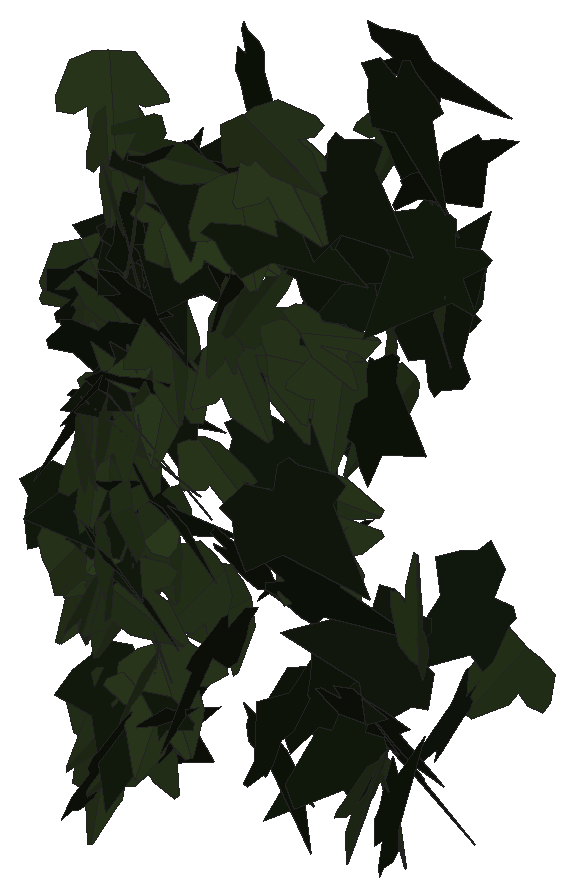
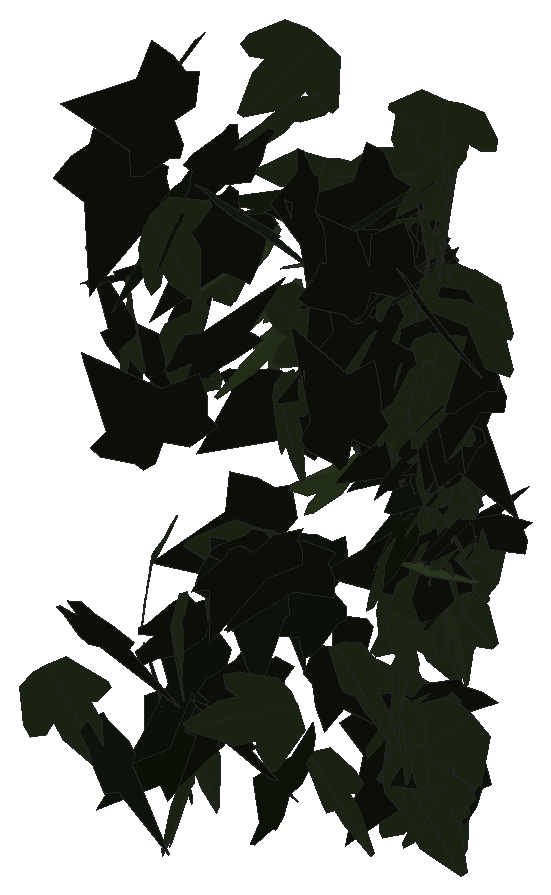
# SketchUp Ruby script. Lengths in inches.
U = 1.inch
M = Sketchup.active_model
def pt(a) = Geom::Point3d.new(a.map { |v| v * U })
def face(e, loops, mat)
  f = e.add_face(loops[0].map { |a| pt(a) })
  loops[1..].each { |l| e.add_face(l.map { |a| pt(a) }).erase! }
  f.material = f.back_material = mat if mat
  f
end
# faces: each face lists its corners as indices into pts; further lists are holes
def faces(e, pts, list, mat = nil) = list.each { |f| face(e, (f[0].is_a?(Array) ? f : [f]).map { |l| l.map { |i| pts[i] } }, mat) }
# xy, xz, yz: faces in a plane at the given z, y or x. An outline is a flat list of corners, or four numbers for a rectangle; further outlines are holes
def ring(l) = l.size == 4 ? [[l[0], l[1]], [l[2], l[1]], [l[2], l[3]], [l[0], l[3]]] : l.each_slice(2).to_a
def flat(e, list, mat, &to3) = list.each { |f| face(e, (f[0].is_a?(Array) ? f : [f]).map { |l| ring(l).map { |u, v| to3.(u, v) } }, mat) }
def xy(e, z, list, mat = nil) = flat(e, list, mat) { |x, y| [x, y, z] }
def xz(e, y, list, mat = nil) = flat(e, list, mat) { |x, z| [x, y, z] }
def yz(e, x, list, mat = nil) = flat(e, list, mat) { |y, z| [x, y, z] }
def lines(e, pts, list) = list.each { |a, b| e.add_line(pt(pts[a]), pt(pts[b])) }
# prism: a flat outline (further loops are holes) pulled along v
def prism(e, loops, v, mat = nil)
  f = face(e, loops, mat); d = Geom::Vector3d.new(v.map { |x| x * U })
  f.pushpull(f.normal.samedirection?(d) ? d.length : -d.length)
end
def box(e, o, s, mat = nil) = prism(e, [[o, [o[0] + s[0], o[1], o[2]], [o[0] + s[0], o[1] + s[1], o[2]], [o[0], o[1] + s[1], o[2]]]], [0, 0, s[2]], mat)
def at(x, y, z, deg = 0) = Geom::Transformation.translation(pt([x, y, z])) * Geom::Transformation.rotation(ORIGIN, Z_AXIS, deg.degrees)
def axes(o, x, y, z) = Geom::Transformation.new([*x, 0, *y, 0, *z, 0, *pt(o).to_a, 1])
def part(name) = M.definitions.add(name)
# library, detail: a bought-in or finely detailed component or shape, given as its bounding box
def library(name, o, s) = part(name).tap { |d| box(d.entities, o, s) }
def detail(e, o, s) = box(e.add_group.entities, o, s)
def put(e, d, t, mat = nil) = e.add_instance(d, t).tap { |i| i.material = mat if mat }
def group(e, t, mat = nil) = e.add_group.tap { |g| g.transformation = t; g.material = mat if mat }.entities
root = M.entities
M.materials.add("efeu1").color = [18, 25, 13]
M.materials.add("efeu2").color = [43, 57, 29]
c1 = part("ivyleaf_10")
p = [[0,0.5,-0.03],[-0.0625,2.02,-0.43],[-0.19,2.01,-0.46],[-0.54,1.05,-0.29],[-0.52,0.625,-0.18],[-0.83,0.76,-0.28],
  [-1.16,0.64,-0.33],[-1.15,0.33,-0.24],[-0.77,-0.39,0.02],[-0.3,-0.51,0.16],[0.04,-0.48,0.23],[-0.02,2.01,-0.4375],
  [-0.06,2.01,-0.43],[0.04,-0.49,0.23],[0.67,-0.49,0.14],[1.38,0.36,-0.2],[1.375,0.51,-0.24],[0.81,0.65,-0.19],
  [0.62,0.59,-0.15],[0.6,1.09,-0.28],[0.5,1.23,-0.31]]
faces(c1.entities,p,[[0,1,2,3,4,5,6,7,8,9,10],[11,12,0,13,14,15,16,17,18,19,20]],"efeu2")
c2 = part("ivyleaf_9")
p = [[1.54,2.16,1.25],[1.36,2.04,1.19],[-0.21,0.99,0.68],[-0.71,1.11,0.82],[-0.85,0.86,0.67],[-0.8,0.17,0.21],
  [-0.9,-0.01,0.1],[-0.67,-0.16,-0.02],[-0.08,-0.08,-0.05],[-0.03,-0.6,-0.4],[0.65,-0.88,-0.66],[0.83,-0.6,-0.49],
  [1.29,-0.42,-0.43],[1.8125,-0.07,-0.26],[1.21,0.44,0.15]]
faces(c2.entities,p,[[0,1,2,3,4,5,6,7,8,9,10,11,12,13,14]],"efeu1")
put(root,c1,axes([46.82,223.79,215.375],[0.30689,-0.17648,-0.35309],[-0.31194,0.16564,-0.35392],[0.24189,0.43752,-0.00843]))
put(root,c2,axes([46.77,221.68,218.99],[-0.26591,0.32248,-0.27441],[0.12873,-0.24713,-0.41516],[-0.40339,-0.29144,0.0484]))
put(root,c1,axes([46.61,221.95,214.38],[0.06345,0.46426,-0.17446],[-0.06333,-0.16686,-0.46706],[-0.4919,0.08136,0.03763]))
put(root,c1,axes([46.6875,221.47,218.47],[-0.1604,0.43532,0.18647],[-0.13321,0.14746,-0.45881],[-0.45445,-0.19687,0.06867]))
put(root,c1,axes([46.83,222.19,214.4375],[0.37847,0.13915,-0.29563],[-0.32579,0.1261,-0.35772],[-0.02499,0.4634,0.18612]))
put(root,c1,axes([46.64,222.06,219.93],[-0.15553,-0.44023,-0.1789],[0.0777,0.16215,-0.46655],[0.4688,-0.17293,0.01797]))
put(root,c1,axes([46.58,221.66,220.17],[-0.44765,-0.1511,-0.16364],[0.16974,0.0064,-0.47026],[0.14421,-0.47658,0.04557]))
put(root,c1,axes([46.58,221.19,217.02],[0.06755,0.12705,-0.47885],[0.14684,0.45643,0.14181],[0.47315,-0.15979,0.02435]))
put(root,c1,axes([46.73,221.78,216.78],[0.16694,0.38069,-0.27786],[-0.18616,-0.21755,-0.4099],[-0.43298,0.24031,0.0691]))
put(root,c2,axes([47.07,221.99,220.55],[-0.28103,0.2768,0.30725],[-0.21871,0.21579,-0.39446],[-0.35098,-0.35611,-0.00021]))
put(root,c1,axes([46.79,221.57,216.68],[0.12726,-0.4742,-0.09455],[-0.03702,0.08792,-0.49081],[0.48211,0.13192,-0.01273]))
put(root,c1,axes([46.6875,221.69,218.05],[0.11882,0.46479,-0.14089],[-0.04843,-0.13298,-0.47955],[-0.48326,0.12761,0.01342]))
put(root,c1,axes([46.78,222.07,219.12],[0.03325,0.46398,-0.18335],[-0.00464,0.18403,0.46488],[0.49887,-0.02921,0.01654]))
put(root,c1,axes([47.08,221.625,217.54],[-0.23958,0.12458,0.42081],[-0.4336,0.00683,-0.24888],[-0.06776,-0.48418,0.10476]))
put(root,c2,axes([46.77,222,217.32],[0.10972,-0.3803,-0.30551],[0.08778,-0.29264,0.3958],[-0.47985,-0.14049,0.00254]))
put(root,c2,axes([46.5,221.61,217.73],[-0.04451,-0.36504,-0.33877],[0.22637,0.28812,-0.34021],[0.44359,-0.18366,0.13962]))
put(root,c2,axes([46.42,221.64,219.87],[0.27297,0.05631,0.41511],[0.3965,0.12515,-0.27771],[-0.13518,0.4808,0.02367]))
put(root,c2,axes([46.79,221.58,219.6],[0.34529,0.32059,-0.16733],[-0.13687,-0.09829,-0.47075],[-0.33473,0.37089,0.01988]))
put(root,c1,axes([46.7,221.54,220.52],[-0.42496,-0.19869,-0.17301],[0.18869,-0.00038,-0.46303],[0.18387,-0.45883,0.0753]))
put(root,c1,axes([46.77,222.03,214.97],[0.01467,-0.18184,0.46553],[0.08905,-0.45733,-0.18144],[0.49179,0.08823,0.01897]))
put(root,c1,axes([46.57,221.89,215.19],[-0.26759,-0.1951,-0.37461],[0.35309,0.14004,-0.32514],[0.23179,-0.43855,0.06283]))
put(root,c1,axes([46.91,222.01,217.02],[0.08621,0.19271,-0.45324],[-0.2035,-0.40508,-0.21094],[-0.4485,0.22084,0.00859]))
put(root,c1,axes([46.77,222.49,216.79],[0.11328,-0.30008,0.38357],[0.11296,-0.36688,-0.32038],[0.47372,0.15924,-0.01533]))
put(root,c1,axes([47.18,221.76,218.17],[0.07671,-0.01508,-0.49385],[-0.44837,0.20781,-0.07599],[0.20755,0.45452,0.01836]))
put(root,c1,axes([46.93,221.7,218.74],[-0.01928,0.46785,0.17534],[-0.18986,0.15545,-0.43565],[-0.46215,-0.08338,0.17166]))
put(root,c2,axes([46.83,222.39,218.76],[0.13338,-0.32118,-0.35924],[0.14471,-0.32884,0.34774],[-0.45964,-0.19674,0.00524]))
put(root,c1,axes([47.04,221.57,218.74],[0.35221,-0.16904,-0.31205],[-0.2773,0.14328,-0.39061],[0.22147,0.44822,0.00718]))
put(root,c1,axes([46.83,221.84,217.07],[0.41424,-0.26825,-0.08031],[0.00776,0.15435,-0.47552],[0.27991,0.39271,0.13203]))
put(root,c1,axes([46.9,222.13,217.24],[-0.49845,-0.02607,0.0295],[0.02483,-0.49892,-0.0214],[0.03055,-0.01987,0.49867]))
put(root,c1,axes([46.96,221.89,216.61],[-0.13131,-0.44619,0.18351],[-0.03547,-0.18074,-0.46484],[0.48115,-0.13509,0.01581]))
put(root,c1,axes([46.98,221.45,221.65],[-0.33317,0.34293,0.1463],[-0.13314,0.07383,-0.47626],[-0.34824,-0.3563,0.04212]))
put(root,c2,axes([46.99,221.2,214.56],[-0.15844,0.29308,-0.37283],[-0.20139,0.3143,0.33265],[0.42934,0.25558,0.01845]))
put(root,c1,axes([47.01,222.17,215.93],[-0.33606,0.34989,0.121],[-0.08049,0.09046,-0.48512],[-0.36136,-0.34554,-0.00447]))
put(root,c1,axes([47.04,222.03,219.15],[0.03664,0.15212,-0.47489],[-0.02414,0.47615,0.15066],[0.49807,0.01189,0.04224]))
put(root,c1,axes([47.12,221.25,216.875],[-0.02583,0.10493,-0.48818],[-0.10809,0.47607,0.10804],[0.48749,0.11112,-0.00191]))
put(root,c1,axes([46.85,221.62,222.72],[0.46319,0.1612,0.09729],[0.08762,0.04414,-0.49028],[-0.16666,0.47124,0.01265]))
put(root,c1,axes([46.93,221.66,222.08],[0.0206,0.47589,-0.15201],[-0.00834,-0.15179,-0.47633],[-0.49951,0.02216,0.00169]))
put(root,c1,axes([47.04,222.14,214.74],[0.01557,-0.25413,0.43032],[0.01222,-0.43021,-0.2545],[0.49961,0.01844,-0.00718]))
put(root,c2,axes([46.63,221.89,217.33],[0.38798,0.01259,0.31514],[0.31157,0.06229,-0.38606],[-0.04898,0.49595,0.04048]))
put(root,c2,axes([46.68,223.57,219.62],[-0.02299,-0.09481,0.49039],[0.36286,-0.34051,-0.04882],[0.34322,0.35364,0.08446]))
put(root,c1,axes([47.25,225.875,217.92],[-0.03166,0.05115,-0.49637],[-0.23881,0.43516,0.06007],[0.43814,0.24088,-0.00313]))
put(root,c1,axes([47.12,222.04,215.56],[0.10552,-0.44612,-0.19962],[-0.05205,0.1928,-0.45839],[0.48596,0.11751,-0.00575]))
put(root,c2,axes([46.71,221.7,217.04],[0.36429,-0.31913,0.1243],[0.09979,-0.07469,-0.48421],[0.32763,0.37759,0.00927]))
put(root,c1,axes([47.22,222.85,216.21],[0.37723,-0.17084,-0.2802],[-0.25699,0.11171,-0.4141],[0.2041,0.45643,-0.00353]))
put(root,c2,axes([46.79,221.62,218.89],[0.44913,0.12155,0.18306],[0.15945,0.10635,-0.46181],[-0.1512,0.4732,0.05676]))
put(root,c1,axes([47.1,221.64,220.94],[-0.29958,0.39759,0.04665],[-0.05124,0.0197,-0.49698],[-0.39702,-0.30255,0.02894]))
put(root,c2,axes([47.07,221.9,215.41],[-0.2799,-0.40493,-0.08769],[0.05211,0.07058,-0.49224],[0.41102,-0.2847,0.00269]))
put(root,c1,axes([47.07,222.01,220.19],[-0.07306,-0.15963,-0.46817],[0.17446,0.43452,-0.17538],[0.46285,-0.18898,-0.0078]))
put(root,c1,axes([46.98,221.58,216.61],[-0.30475,-0.20215,-0.34097],[0.30985,0.14677,-0.36394],[0.24723,-0.43312,0.03582]))
put(root,c1,axes([46.99,221.84,221.42],[0.3706,-0.23549,0.23916],[0.20527,-0.12286,-0.43906],[0.26555,0.42361,0.00561]))
put(root,c2,axes([46.91,222.16,217.81],[0.38681,-0.31542,0.02987],[0.01646,-0.02706,-0.499],[0.3164,0.38701,-0.01055]))
put(root,c1,axes([46.89,224.65,216.54],[-0.16502,-0.06552,-0.46741],[0.45476,0.11048,-0.17604],[0.12635,-0.48322,0.02313]))
put(root,c2,axes([47.0625,221.99,220.71],[0.08964,-0.44345,-0.21287],[-0.04873,0.20731,-0.45238],[0.48948,0.10185,-0.00606]))
put(root,c1,axes([47.13,222.1875,217.26],[0.01903,-0.49963,0.00328],[0.18506,0.004,-0.46447],[0.4641,0.01889,0.18508]))
put(root,c2,axes([47.1875,221.74,214.79],[0.25418,0.40568,0.14428],[0.07424,0.12374,-0.47872],[-0.42413,0.26478,0.00267]))
put(root,c2,axes([47.03,221.4,220.34],[0.49698,0.04863,-0.02548],[-0.02536,-0.00248,-0.49935],[-0.04869,0.49762,0]))
put(root,c2,axes([46.84,221.84,218.34],[0.21613,-0.31536,0.32223],[0.30304,-0.16299,-0.36277],[0.33385,0.35211,0.12068]))
put(root,c1,axes([47.28,222.13,219.25],[0.11303,-0.48643,-0.0247],[-0.00136,0.02504,-0.49937],[0.48705,0.11295,0.00434]))
put(root,c2,axes([47.21,221.77,220.65],[-0.06908,-0.11012,0.48281],[0.27459,0.39716,0.12987],[-0.4121,0.28309,0.0056]))
put(root,c2,axes([47.11,222.17,219.19],[0.06506,-0.4642,-0.17402],[-0.02469,0.17226,-0.46874],[0.49513,0.06959,-0.00051]))
put(root,c2,axes([46.99,222.53,220.21],[0.47448,0.05094,0.14923],[0.1496,0.00416,-0.47708],[-0.04985,0.49738,-0.01129]))
put(root,c1,axes([47.22,222.08,215.13],[-0.24468,-0.26366,0.34729],[0.23603,-0.41494,-0.14872],[0.36663,0.09117,0.32752]))
put(root,c2,axes([47.0625,221.62,218.72],[0.46036,-0.19434,0.0175],[0.01655,-0.0058,-0.49969],[0.19442,0.46065,0.00109]))
put(root,c2,axes([47.2,224.62,218.36],[0.04208,-0.42382,-0.26193],[-0.02957,0.26028,-0.42589],[0.49735,0.05133,-0.00316]))
put(root,c2,axes([47.18,221.76,221.01],[0.04444,0.03877,-0.49651],[0.05402,0.49517,0.0435],[0.49508,-0.0575,0.03982]))
put(root,c1,axes([47.29,222.09,219.07],[-0.24222,-0.35782,0.25159],[0.23431,-0.34899,-0.27076],[0.36937,-0.01327,0.33674]))
put(root,c2,axes([47.21,222.58,220.84],[-0.15698,-0.07507,0.46874],[0.46812,0.05757,0.16599],[-0.0789,0.49097,0.05221]))
put(root,c1,axes([47.33,222.2,221.1],[-0.13752,-0.38235,0.29136],[0.19858,-0.32117,-0.32774],[0.43778,0.02557,0.24019]))
put(root,c1,axes([47.25,222,215.55],[0.38898,0.24821,0.19258],[0.16302,0.10252,-0.46143],[-0.26855,0.42176,-0.00118]))
put(root,c2,axes([47.23,222.18,221.67],[0.01862,-0.48418,0.12339],[0.18798,-0.10762,-0.45064],[0.46294,0.06318,0.17803]))
put(root,c2,axes([47.31,222.19,220.52],[-0.13756,-0.38111,0.29297],[0.19861,-0.32256,-0.32635],[0.43776,0.02659,0.24013]))
put(root,c1,axes([47.17,221.66,221.87],[0.09736,-0.08169,0.48358],[0.39188,0.30939,-0.02664],[-0.29488,0.38419,0.12427]))
put(root,c1,axes([47.39,221.97,219.68],[-0.01774,-0.48976,0.09909],[0.23773,-0.09548,-0.42938],[0.43951,0.03187,0.23625]))
put(root,c2,axes([47.23,223.51,222.21],[0.04571,-0.04238,-0.4961],[0.4979,0.00138,0.04576],[-0.00251,-0.4982,0.04233]))
put(root,c2,axes([47.25,221.99,221.42],[0.29116,0.01323,0.40626],[0.39058,0.1293,-0.28413],[-0.11258,0.48281,0.06496]))
put(root,c2,axes([47.81,222.41,215.98],[-0.2064,0.24126,-0.38626],[0.22689,-0.31322,-0.31688],[-0.39487,-0.30608,0.01982]))
put(root,c2,axes([47.62,223.65,217.83],[-0.1407,-0.30014,-0.37433],[0.18129,0.32792,-0.33107],[0.44423,-0.22888,0.01655]))
put(root,c1,axes([48.05,222.98,219.28],[0.24265,-0.13176,-0.41685],[-0.25565,0.34397,-0.25754],[0.35463,0.33812,0.09956]))
put(root,c2,axes([48.09,222.15,220.47],[-0.06248,0.05533,-0.49299],[-0.40006,0.28819,0.08305],[0.29333,0.40483,0.00826]))
put(root,c1,axes([47.6,222.2,220.95],[0.01227,-0.46926,-0.17219],[0.48721,0.04972,-0.10078],[0.11171,-0.16531,0.45847]))
put(root,c2,axes([47.75,222.61,216.83],[0.45259,-0.14414,0.15615],[0.15186,-0.03763,-0.47489],[0.14865,0.47729,0.00972]))
put(root,c1,axes([47.76,222.21,218.16],[0.01257,-0.48045,0.13789],[0.47466,-0.03175,-0.15391],[0.15664,0.13477,0.4553]))
put(root,c1,axes([48.02,222.13,220.03],[0.17632,-0.45132,-0.12337],[0.18391,0.18808,-0.42521],[0.43022,0.10457,0.23232]))
put(root,c1,axes([48.1875,222.3,219.89],[0.07391,-0.3486,0.35074],[-0.0323,0.35047,0.35514],[-0.49345,-0.07515,0.02928]))
put(root,c2,axes([47.98,223.03,214.38],[0.19721,-0.37847,0.26051],[0.11927,-0.2316,-0.42677],[0.44371,0.23047,-0.00107]))
put(root,c1,axes([48.11,222.14,219.55],[-0.04019,-0.49416,-0.06472],[0.29038,0.02955,-0.40596],[0.40505,-0.07022,0.28462]))
put(root,c2,axes([48.56,222.91,216.94],[-0.00826,0.49786,0.04549],[-0.05292,0.04437,-0.49521],[-0.49712,-0.013,0.05196]))
put(root,c2,axes([48.66,223.77,219.95],[-0.19056,-0.46213,-0.01088],[0.02162,-0.02066,0.4991],[-0.46176,0.18975,0.02786]))
put(root,c1,axes([48.35,221.96,221.63],[0.38569,0.30027,0.10529],[0.08563,0.06141,-0.48877],[-0.30645,0.39506,-0.00406]))
put(root,c2,axes([48.99,222.73,221.29],[-0.3453,0.30435,0.1953],[-0.2382,0.01175,-0.43946],[-0.27208,-0.39653,0.13687]))
put(root,c2,axes([48.59,222.91,215.6],[0.08199,-0.19323,-0.45381],[-0.16923,0.42109,-0.20987],[0.46329,0.18801,0.00365]))
put(root,c1,axes([48.71,224.31,221.75],[-0.00068,-0.44602,0.22597],[0.03043,-0.22559,-0.44518],[0.49907,0.01315,0.02745]))
put(root,c2,axes([48.42,222.11,221.34],[0.29965,-0.38805,-0.09811],[0.24521,0.27484,-0.33813],[0.31635,0.15453,0.35502]))
put(root,c1,axes([48.71,222.78,217.16],[0.24543,0.37475,0.22209],[0.07541,0.21451,-0.44531],[-0.42904,0.25208,0.04878]))
put(root,c2,axes([48.68,224.39,219.23],[-0.18449,-0.06929,0.45953],[0.45276,0.08465,0.19453],[-0.10476,0.48789,0.03151]))
put(root,c2,axes([49.13,223.02,214.96],[-0.49725,0.0511,-0.01161],[0.00874,-0.0283,-0.49912],[-0.05167,-0.49658,0.02725]))
put(root,c2,axes([48.82,223.96,221.78],[0.39067,-0.25674,-0.17738],[-0.14876,0.09661,-0.46748],[0.27431,0.41803,-0.00091]))
put(root,c1,axes([48.81,222.06,219.48],[0.37727,-0.28697,-0.15911],[0.2235,0.40225,-0.19555],[0.24024,0.07643,0.43179]))
put(root,c1,axes([48.89,221.64,222.79],[-0.38191,-0.13176,-0.29459],[0.28208,0.08543,-0.4039],[0.15677,-0.4747,0.00908]))
put(root,c1,axes([48.81,222.03,222.22],[-0.09518,-0.4895,-0.03644],[0.38505,-0.05143,-0.31479],[0.30443,-0.08798,0.38676]))
put(root,c1,axes([48.9,221.98,219.85],[0.31657,-0.27043,-0.27685],[0.21911,0.42007,-0.15979],[0.31902,-0.02015,0.38447]))
put(root,c2,axes([49.02,222.65,221.1],[0.04337,-0.07492,-0.49245],[-0.15777,0.4668,-0.08491],[0.47247,0.16275,0.01685]))
put(root,c2,axes([48.77,222.29,216.99],[0.41609,-0.01093,0.27704],[0.27627,-0.02581,-0.41594],[0.0234,0.49921,-0.01544]))
put(root,c2,axes([49.44,221.29,215.78],[-0.14333,0.36068,0.31523],[-0.12309,0.29026,-0.38807],[-0.46293,-0.18885,0.00559]))
put(root,c1,axes([49.09,223.47,214.26],[-0.28742,0.3954,-0.10511],[0.07029,-0.07882,-0.48872],[-0.40305,-0.29572,-0.01028]))
put(root,c2,axes([49.14,222.5,221.93],[0.15935,-0.228,-0.41548],[-0.13829,0.39689,-0.27084],[0.4533,0.20123,0.06343]))
put(root,c2,axes([49.07,222.88,215.38],[0.49932,0.02543,0.00573],[0.00493,0.01588,-0.49972],[-0.02559,0.4991,0.01561]))
put(root,c2,axes([49.55,223.3,215.97],[-0.05573,-0.41248,-0.27704],[-0.04375,-0.27362,0.41619],[-0.49495,0.07063,-0.00559]))
put(root,c2,axes([49.08,221.68,218.41],[-0.03009,-0.17822,-0.46619],[0.27041,0.38672,-0.1653],[0.41949,-0.26207,0.07311]))
put(root,c2,axes([49.6,224.23,215.02],[-0.35976,0.32903,-0.11093],[0.07741,-0.07972,-0.4875],[-0.33849,-0.36794,0.00641]))
put(root,c1,axes([49.41,222.875,214.6],[0.13436,-0.47353,0.08782],[0.0255,-0.08405,-0.49222],[0.48093,0.13675,0.00157]))
put(root,c2,axes([49.1,223.71,222.79],[0.33814,-0.14506,0.33855],[0.31707,-0.11922,-0.36777],[0.18742,0.4634,0.01136]))
put(root,c2,axes([49.27,223.3,214.82],[0.47514,-0.15448,-0.01949],[-0.01918,0.00405,-0.49962],[0.15452,0.47552,-0.00208]))
put(root,c1,axes([49.4375,221.85,220.38],[0.42887,-0.17085,-0.19205],[0.13526,0.46767,-0.11399],[0.21858,0.04582,0.44735]))
put(root,c1,axes([49.89,223.47,219.94],[-0.0332,0.01799,0.49857],[-0.4396,0.23522,-0.03776],[-0.23591,-0.44085,0.0002]))
put(root,c2,axes([49.72,223.8,220.67],[-0.34642,-0.32083,0.16449],[0.00185,-0.22969,-0.44411],[0.36054,-0.30709,0.16033]))
put(root,c1,axes([49.68,222.97,219.26],[0.02684,-0.30135,0.39808],[0.06933,-0.39254,-0.30183],[0.49444,0.0714,0.02072]))
put(root,c2,axes([49.96,224.15,216.38],[-0.49604,0.04407,0.04478],[-0.04444,0.00586,-0.49799],[-0.04442,-0.49802,-0.0019]))
put(root,c2,axes([49.8,223.52,221.8],[0.17311,0.46617,0.05215],[0.0283,0.04511,-0.49716],[-0.46822,0.17508,-0.01077]))
put(root,c2,axes([49.55,223.14,222.9],[0.24301,-0.43596,-0.02971],[-0.01432,0.02604,-0.49912],[0.43674,0.24343,0.00017]))
put(root,c2,axes([49.6,223.58,219.46],[-0.20419,0.20996,0.40525],[0.26218,-0.30944,0.29242],[0.37359,0.33191,0.01627]))
put(root,c2,axes([49.67,222.76,214.04],[-0.14048,0.35158,0.32659],[0.06602,-0.3229,0.376],[0.4753,0.14876,0.0443]))
put(root,c1,axes([50.01,222.82,216.45],[-0.05135,0.29444,-0.40083],[-0.14443,0.37677,0.29527],[0.47592,0.14611,0.04635]))
put(root,c1,axes([50.12,224.43,215.59],[-0.38408,-0.08848,0.30766],[-0.2765,-0.15048,-0.38846],[0.16133,-0.46854,0.06667]))
put(root,c1,axes([49.75,221.9375,219.98],[-0.14391,-0.41475,0.23931],[0.22967,-0.27905,-0.34552],[0.42017,0.01048,0.27083]))
put(root,c2,axes([49.9,222.23,219.61],[0.16887,-0.12016,-0.45502],[-0.32556,0.31926,-0.20514],[0.33984,0.36556,0.02959]))
